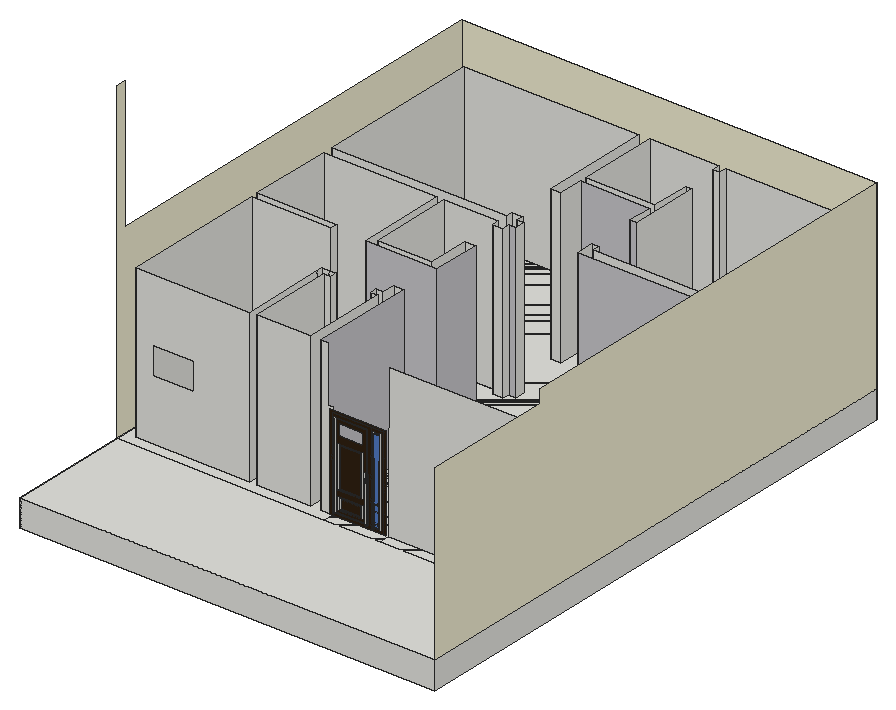
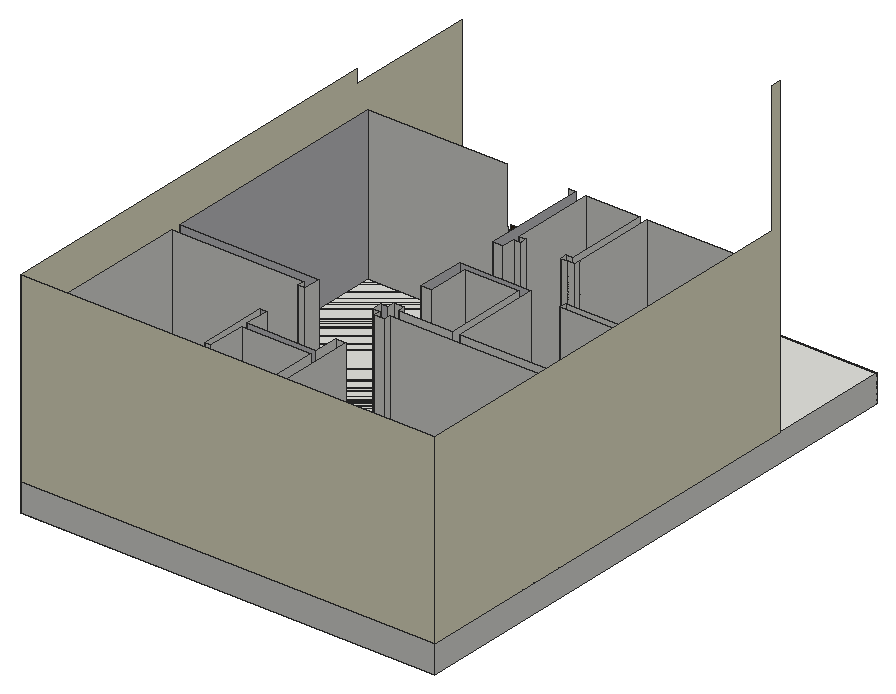
# SketchUp Ruby script. Lengths in inches.
U = 1.inch
M = Sketchup.active_model
def pt(a) = Geom::Point3d.new(a.map { |v| v * U })
def face(e, loops, mat)
  f = e.add_face(loops[0].map { |a| pt(a) })
  loops[1..].each { |l| e.add_face(l.map { |a| pt(a) }).erase! }
  f.material = f.back_material = mat if mat
  f
end
# faces: each face lists its corners as indices into pts; further lists are holes
def faces(e, pts, list, mat = nil) = list.each { |f| face(e, (f[0].is_a?(Array) ? f : [f]).map { |l| l.map { |i| pts[i] } }, mat) }
# xy, xz, yz: faces in a plane at the given z, y or x. An outline is a flat list of corners, or four numbers for a rectangle; further outlines are holes
def ring(l) = l.size == 4 ? [[l[0], l[1]], [l[2], l[1]], [l[2], l[3]], [l[0], l[3]]] : l.each_slice(2).to_a
def flat(e, list, mat, &to3) = list.each { |f| face(e, (f[0].is_a?(Array) ? f : [f]).map { |l| ring(l).map { |u, v| to3.(u, v) } }, mat) }
def xy(e, z, list, mat = nil) = flat(e, list, mat) { |x, y| [x, y, z] }
def xz(e, y, list, mat = nil) = flat(e, list, mat) { |x, z| [x, y, z] }
def yz(e, x, list, mat = nil) = flat(e, list, mat) { |y, z| [x, y, z] }
def lines(e, pts, list) = list.each { |a, b| e.add_line(pt(pts[a]), pt(pts[b])) }
# prism: a flat outline (further loops are holes) pulled along v
def prism(e, loops, v, mat = nil)
  f = face(e, loops, mat); d = Geom::Vector3d.new(v.map { |x| x * U })
  f.pushpull(f.normal.samedirection?(d) ? d.length : -d.length)
end
def box(e, o, s, mat = nil) = prism(e, [[o, [o[0] + s[0], o[1], o[2]], [o[0] + s[0], o[1] + s[1], o[2]], [o[0], o[1] + s[1], o[2]]]], [0, 0, s[2]], mat)
def at(x, y, z, deg = 0) = Geom::Transformation.translation(pt([x, y, z])) * Geom::Transformation.rotation(ORIGIN, Z_AXIS, deg.degrees)
def axes(o, x, y, z) = Geom::Transformation.new([*x, 0, *y, 0, *z, 0, *pt(o).to_a, 1])
def part(name) = M.definitions.add(name)
# library, detail: a bought-in or finely detailed component or shape, given as its bounding box
def library(name, o, s) = part(name).tap { |d| box(d.entities, o, s) }
def detail(e, o, s) = box(e.add_group.entities, o, s)
def put(e, d, t, mat = nil) = e.add_instance(d, t).tap { |i| i.material = mat if mat }
def group(e, t, mat = nil) = e.add_group.tap { |g| g.transformation = t; g.material = mat if mat }.entities
root = M.entities
M.materials.add("Lily_Blonde").color = [237, 233, 206]
M.materials.add("Panel-Opening1").color = [191, 148, 107]
M.materials.add("Stained Mahogany").color = [48, 33, 18]
M.materials.add("[Aluminum]").color = [178, 178, 178]
M.materials.add("[Metal Rusted]").color = [181, 73, 64]
M.materials.add("[Metal Silver]").color = [198, 197, 201]
M.materials.add("[Translucent Glass Blue]").color = [81, 121, 193]
c1 = part("A$C72384DA6")
p = [[1968.53,82677.18,0],[49212.62,82677.18,0],[0.02,84645.6875,0],[51181.125,84645.6875,0],[49212.62,0.02,0],[51181.125,0.02,0],
  [1968.53,0.02,0],[0.02,0.02,0]]
lines(c1.entities,p,[[0,1],[2,3],[1,4],[3,5],[0,6],[2,7],[7,6],[4,5]])
c2 = part("Floor slab")
box(c2.entities,[0,0,0],[360,480,24])
xy(root,24,[[0,125.1875,0,500.1875,360,500.1875,360,125.1875,229,125.1875,229,134.1875,351,134.1875,351,338.1875,230,338.1875,230,353.1875,236,353.1875,236,347.1875,351,347.1875,351,491.1875,236,491.1875,236,485.1875,230,485.1875,230,491.1875,170,491.1875,170,422.1875,230,422.1875,230,455.1875,236,455.1875,236,395.1875,230,395.1875,230,416.1875,170,416.1875,170,395.1875,161,395.1875,161,491.1875,9,491.1875,9,347.1875,161,347.1875,161,353.1875,170,353.1875,170,347.1875,176,347.1875,176,338.1875,170,338.1875,170,332.1875,161,332.1875,161,338.1875,114,338.1875,114,266.1875,161,266.1875,161,302.1875,170,302.1875,170,260.1875,108,260.1875,108,338.1875,9,338.1875,9,266.1875,78,266.1875,78,260.1875,9,260.1875,9,134.1875,108,134.1875,108,213.1875,120,213.1875,120,207.1875,114,207.1875,114,134.1875,161,134.1875,161,207.1875,155,207.1875,155,213.1875,161,213.1875,161,224.1875,170,224.1875,170,134.1875,180.027,134.1875,180.027,125.1875],[180.027,125.1875,180.027,134.1875,170,134.1875,170,224.1875,161,224.1875,161,213.1875,155,213.1875,155,207.1875,161,207.1875,161,134.1875,114,134.1875,114,207.1875,120,207.1875,120,213.1875,108,213.1875,108,134.1875,9,134.1875,9,260.1875,78,260.1875,78,266.1875,9,266.1875,9,338.1875,108,338.1875,108,260.1875,170,260.1875,170,302.1875,161,302.1875,161,266.1875,114,266.1875,114,338.1875,161,338.1875,161,332.1875,170,332.1875,170,338.1875,176,338.1875,176,347.1875,170,347.1875,170,353.1875,161,353.1875,161,347.1875,9,347.1875,9,491.1875,161,491.1875,161,395.1875,170,395.1875,170,416.1875,230,416.1875,230,395.1875,236,395.1875,236,455.1875,230,455.1875,230,422.1875,170,422.1875,170,491.1875,230,491.1875,230,485.1875,236,485.1875,236,491.1875,351,491.1875,351,347.1875,236,347.1875,236,353.1875,230,353.1875,230,338.1875,351,338.1875,351,134.1875,229,134.1875,229,125.1875]])
xy(root,28.183,[[218.2,130.405,224.188,131.153]])
xy(root,28.183,[[184.518,131.153,212.961,131.528],[218.2,131.153,224.188,131.528]],"Panel-Opening1")
xy(root,29.332,[[185.641,130.031,211.838,131.153]])
xy(root,29.332,[[219.323,130.592,223.066,131.528],[185.641,131.153,211.838,131.528]],"Panel-Opening1")
xy(root,32.204,[[188.447,130.031,209.031,131.153]])
xy(root,32.204,[[219.323,130.031,223.066,131.528],[188.447,131.153,209.031,131.528]],"Panel-Opening1")
xy(root,33.353,[[189.57,130.405,207.909,131.153]])
xy(root,33.353,[[219.323,130.031,223.066,131.528],[189.57,131.153,207.909,131.528]],"Panel-Opening1")
xy(root,41.012,[[189.57,130.405,207.909,131.153]])
xy(root,41.012,[[219.323,130.031,223.066,131.528],[189.57,131.153,207.909,131.528]],"Panel-Opening1")
xy(root,42.135,[[219.323,130.031,223.066,131.528]],"Panel-Opening1")
xy(root,42.161,[[188.447,130.031,209.031,131.153]])
xy(root,42.161,[[188.447,131.153,209.031,131.528]],"Panel-Opening1")
xy(root,47.905,[[188.447,130.031,209.031,131.153]])
xy(root,47.905,[[219.323,130.031,223.066,131.528],[188.447,131.153,209.031,131.528]],"Panel-Opening1")
xy(root,49.054,[[189.57,130.405,207.909,131.153]])
xy(root,49.054,[[219.323,130.031,223.066,131.528],[189.57,131.153,207.909,131.528]],"Panel-Opening1")
xy(root,61.961,[[211.838,129.656,212.961,131.528],[210.464,130.031,211.838,131.153]])
xy(root,61.961,[[210.464,131.153,211.838,131.528]],"[Aluminum]")
xy(root,62.37,[[211.693,131.528,211.713,131.715],[211.713,131.528,211.733,131.715]],"[Aluminum]")
xy(root,64.162,[[211.701,129.095,211.705,131.715],[211.721,129.095,211.724,131.715]],"[Metal Rusted]")
xy(root,64.163,[[211.709,129.095,211.713,131.715],[211.713,129.095,211.717,131.715]],"[Metal Rusted]")
xz(root,130.405,[[189.57,49.054,207.909,82.371]],"Stained Mahogany")
xz(root,130.592,[[219.323,29.332,223.066,102.093]],"[Translucent Glass Blue]")
xz(root,131.153,[[180.027,25.502,180.027,107.838,228.68,107.838,228.68,25.502,226.808,25.502,226.808,105.923,181.898,105.923,181.898,25.502],[[181.898,25.502,215.581,105.923],[184.518,28.183,212.961,103.242]],[[215.581,25.502,226.808,105.923],[218.2,28.183,224.188,103.242]],[[185.641,29.332,185.641,102.093,211.838,102.093,211.838,68.107,210.464,68.107,210.464,61.961,211.838,61.961,211.838,29.332],[188.447,47.905,209.031,83.52],[188.447,89.264,209.031,99.221],[188.447,32.204,209.031,42.161]],[189.57,33.353,207.909,41.012],
  [189.57,49.054,207.909,82.371]],"Stained Mahogany")
xz(root,131.528,[[184.518,28.183,184.518,103.242,212.961,103.242,212.961,68.107,211.838,68.107,211.838,102.093,185.641,102.093,185.641,29.332,211.838,29.332,211.838,61.961,212.961,61.961,212.961,28.183],[[218.2,28.183,224.188,103.242],[219.323,49.054,223.066,82.371],[219.323,33.353,223.066,41.012],[219.323,90.413,223.066,98.072],[219.323,42.135,223.066,47.905],[219.323,83.52,223.066,89.264],[219.323,99.221,223.066,102.093],[219.323,29.332,223.066,32.204]],[[188.447,32.204,209.031,42.161],[189.57,33.353,207.909,41.012]],[[188.447,47.905,209.031,83.52],[189.57,49.054,207.909,82.371]]],"Panel-Opening1")
xz(root,131.528,[[[210.464,61.961,212.961,68.107],[211.713,65.58,211.776,65.583,211.838,65.589,211.9,65.599,211.961,65.614,212.022,65.633,212.081,65.655,212.138,65.682,212.193,65.712,212.247,65.746,212.298,65.784,212.347,65.825,212.392,65.869,212.435,65.916,212.475,65.965,212.512,66.018,212.545,66.072,212.575,66.129,212.601,66.188,212.623,66.248,212.641,66.31,212.656,66.372,212.666,66.436,212.672,66.5,212.674,66.564,212.672,66.629,212.666,66.693,212.656,66.756,212.641,66.819,212.623,66.88,212.601,66.941,212.575,66.999,212.545,67.056,212.512,67.111,212.475,67.163,212.435,67.213,212.392,67.26,212.347,67.304,212.298,67.345,212.247,67.382,212.193,67.416,212.138,67.447,212.081,67.473,212.022,67.496,211.961,67.514,211.9,67.529,211.838,67.54,211.776,67.546,211.713,67.548,211.65,67.546,211.587,67.54,211.525,67.529,211.464,67.514,211.404,67.496,211.345,67.473,211.287,67.447,211.232,67.416,211.179,67.382,211.127,67.345,211.079,67.304,211.033,67.26,210.99,67.213,210.95,67.163,210.913,67.111,210.88,67.056,210.85,66.999,210.824,66.941,210.802,66.88,210.784,66.819,210.77,66.756,210.759,66.693,210.753,66.629,210.751,66.564,210.753,66.5,210.759,66.436,210.77,66.372,210.784,66.31,210.802,66.248,210.824,66.188,210.85,66.129,210.88,66.072,210.913,66.018,210.95,65.965,210.99,65.916,211.033,65.869,211.079,65.825,211.127,65.784,211.179,65.746,211.232,65.712,211.287,65.682,211.345,65.655,211.404,65.633,211.464,65.614,211.525,65.599,211.587,65.589,211.65,65.583],[211.693,62.37,211.733,62.37,211.753,62.372,211.773,62.376,211.792,62.38,211.811,62.386,211.83,62.394,211.838,62.397,211.849,62.402,211.866,62.412,211.883,62.423,211.9,62.435,211.915,62.448,211.93,62.462,211.944,62.477,211.968,62.509,211.979,62.527,211.988,62.545,211.997,62.564,212.004,62.583,212.014,62.623,212.017,62.643,212.019,62.664,212.02,62.684,212.02,64.101,212.019,64.122,212.017,64.142,212.014,64.163,212.004,64.203,211.997,64.222,211.988,64.241,211.979,64.259,211.968,64.276,211.956,64.293,211.944,64.309,211.93,64.324,211.915,64.338,211.9,64.351,211.883,64.363,211.866,64.374,211.849,64.383,211.838,64.388,211.83,64.392,211.811,64.399,211.792,64.405,211.773,64.41,211.753,64.413,211.733,64.415,211.713,64.416,211.693,64.415,211.673,64.413,211.653,64.41,211.633,64.405,211.614,64.399,211.595,64.392,211.559,64.374,211.542,64.363,211.526,64.351,211.51,64.338,211.495,64.324,211.482,64.309,211.469,64.293,211.457,64.276,211.447,64.259,211.437,64.241,211.429,64.222,211.422,64.203,211.416,64.183,211.411,64.163,211.408,64.142,211.406,64.122,211.405,64.101,211.405,62.684,211.406,62.664,211.408,62.643,211.411,62.623,211.416,62.603,211.422,62.583,211.429,62.564,211.437,62.545,211.457,62.509,211.469,62.493,211.482,62.477,211.495,62.462,211.51,62.448,211.526,62.435,211.542,62.423,211.559,62.412,211.577,62.402,211.595,62.394,211.614,62.386,211.633,62.38,211.673,62.372]]],"[Aluminum]")
xz(root,131.715,[[[211.693,62.37,211.673,62.372,211.633,62.38,211.614,62.386,211.595,62.394,211.577,62.402,211.559,62.412,211.542,62.423,211.526,62.435,211.51,62.448,211.495,62.462,211.482,62.477,211.469,62.493,211.457,62.509,211.437,62.545,211.429,62.564,211.422,62.583,211.416,62.603,211.411,62.623,211.408,62.643,211.406,62.664,211.405,62.684,211.405,64.101,211.406,64.122,211.408,64.142,211.411,64.163,211.416,64.183,211.422,64.203,211.429,64.222,211.437,64.241,211.447,64.259,211.457,64.276,211.469,64.293,211.482,64.309,211.495,64.324,211.51,64.338,211.526,64.351,211.542,64.363,211.559,64.374,211.595,64.392,211.614,64.399,211.633,64.405,211.653,64.41,211.673,64.413,211.693,64.415,211.713,64.416,211.733,64.415,211.753,64.413,211.773,64.41,211.792,64.405,211.811,64.399,211.83,64.392,211.838,64.388,211.849,64.383,211.866,64.374,211.883,64.363,211.9,64.351,211.915,64.338,211.93,64.324,211.944,64.309,211.956,64.293,211.968,64.276,211.979,64.259,211.988,64.241,211.997,64.222,212.004,64.203,212.014,64.163,212.017,64.142,212.019,64.122,212.02,64.101,212.02,62.684,212.019,62.664,212.017,62.643,212.014,62.623,212.004,62.583,211.997,62.564,211.988,62.545,211.979,62.527,211.968,62.509,211.944,62.477,211.93,62.462,211.915,62.448,211.9,62.435,211.883,62.423,211.866,62.412,211.849,62.402,211.838,62.397,211.83,62.394,211.811,62.386,211.792,62.38,211.773,62.376,211.753,62.372,211.733,62.37],[211.652,62.916,211.773,62.916,211.773,64.105,211.772,64.109,211.772,64.113,211.77,64.121,211.768,64.125,211.767,64.128,211.765,64.132,211.763,64.135,211.761,64.139,211.75,64.15,211.746,64.152,211.743,64.154,211.739,64.156,211.736,64.158,211.732,64.159,211.728,64.161,211.724,64.162,211.721,64.162,211.717,64.163,211.709,64.163,211.705,64.162,211.701,64.162,211.697,64.161,211.693,64.159,211.689,64.158,211.686,64.156,211.682,64.154,211.676,64.15,211.673,64.147,211.67,64.145,211.667,64.142,211.665,64.139,211.662,64.135,211.66,64.132,211.658,64.128,211.657,64.125,211.655,64.121,211.653,64.113,211.653,64.109,211.652,64.105]]],"[Aluminum]")
xz(root,134.1875,[[[9,24,108,156],[24,77,60,101]],[114,24,161,156],[170,24,170,156,176,156,176,108,180.027,108,180.027,24],[229,24,229,108,230,108,230,156,351,156,351,24]])
xz(root,207.1875,[[114,24,120,156],[155,24,161,156]])
xz(root,213.1875,[[108,24,114,156],[114,24,120,156],[155,24,161,156]])
xz(root,224.1875,[[161,24,170,156]])
xz(root,260.1875,[[9,24,78,156]])
xz(root,260.1875,[[108,24,170,156]],"[Metal Silver]")
xz(root,266.1875,[[9,24,78,156],[114,24,161,156]])
xz(root,302.1875,[[161,24,170,156]])
xz(root,332.1875,[[161,24,170,156]])
xz(root,338.1875,[[9,24,108,156],[114,24,161,156]])
xz(root,338.1875,[[170,24,176,156],[230,24,351,156]],"[Metal Silver]")
xz(root,347.1875,[[9,24,161,156],[170,24,176,156],[236,24,351,156]])
xz(root,353.1875,[[161,24,170,156],[230,24,236,156]])
xz(root,395.1875,[[161,24,170,156]])
xz(root,395.1875,[[230,24,236,156]],"[Metal Silver]")
xz(root,416.1875,[[170,24,230,156]],"[Metal Silver]")
xz(root,422.1875,[[170,24,230,156]])
xz(root,455.1875,[[230,24,236,156]])
xz(root,485.1875,[[230,24,236,156]])
xz(root,491.1875,[[9,24,161,156],[170,24,230,156],[236,24,351,156]])
xz(root,500.1875,[[0,24,360,185]],"Lily_Blonde")
yz(root,0,[[125.1875,24,125.1875,298,134.1875,298,134.1875,185,500.1875,185,500.1875,24]],"Lily_Blonde")
yz(root,9,[[134.1875,24,260.1875,156],[266.1875,24,338.1875,156],[347.1875,24,491.1875,156]])
yz(root,78,[[260.1875,24,266.1875,156]])
yz(root,108,[[134.1875,24,207.1875,156],[207.1875,24,213.1875,156],[260.1875,24,338.1875,156]])
yz(root,114,[[134.1875,24,207.1875,156],[266.1875,24,338.1875,156]])
yz(root,120,[[207.1875,24,213.1875,156]])
yz(root,155,[[207.1875,24,213.1875,156]])
yz(root,161,[[134.1875,24,207.1875,156],[213.1875,24,224.1875,156],[266.1875,24,302.1875,156],[332.1875,24,338.1875,156],[347.1875,24,353.1875,156],
  [395.1875,24,491.1875,156]])
yz(root,170,[[332.1875,24,338.1875,156],[347.1875,24,353.1875,156],[395.1875,24,416.1875,156],[422.1875,24,491.1875,156]])
yz(root,170,[[134.1875,24,224.1875,156],[260.1875,24,302.1875,156]],"[Metal Silver]")
yz(root,176,[[338.1875,24,347.1875,156]])
yz(root,184.518,[[129.656,28.183,131.153,103.242]])
yz(root,184.518,[[131.153,28.183,131.528,103.242]],"Panel-Opening1")
yz(root,185.641,[[130.031,29.332,131.153,102.093]])
yz(root,185.641,[[131.153,29.332,131.528,102.093]],"Panel-Opening1")
yz(root,188.447,[[130.031,32.204,131.153,42.161],[130.031,47.905,131.153,83.52]])
yz(root,188.447,[[131.153,32.204,131.528,42.161],[131.153,47.905,131.528,83.52]],"Panel-Opening1")
yz(root,189.57,[[130.405,33.353,131.153,41.012],[130.405,49.054,131.153,82.371]])
yz(root,189.57,[[131.153,33.353,131.528,41.012],[131.153,49.054,131.528,82.371]],"Panel-Opening1")
yz(root,207.909,[[130.405,33.353,131.153,41.012],[130.405,49.054,131.153,82.371]])
yz(root,207.909,[[131.153,33.353,131.528,41.012],[131.153,49.054,131.528,82.371]],"Panel-Opening1")
yz(root,209.031,[[130.031,32.204,131.153,42.161],[130.031,47.905,131.153,83.52]])
yz(root,209.031,[[131.153,32.204,131.528,42.161],[131.153,47.905,131.528,83.52]],"Panel-Opening1")
yz(root,210.464,[[130.031,61.961,131.153,68.107]])
yz(root,210.464,[[131.153,61.961,131.528,68.107]],"[Aluminum]")
yz(root,211.405,[[131.528,62.684,131.715,64.101]],"[Aluminum]")
yz(root,211.838,[[130.031,29.332,131.153,61.961]])
yz(root,211.838,[[131.153,29.332,131.528,61.961]],"Panel-Opening1")
yz(root,212.02,[[131.528,62.684,131.715,64.101]],"[Aluminum]")
yz(root,212.961,[[131.153,28.183,131.528,61.961]],"Panel-Opening1")
yz(root,212.961,[[131.153,61.961,131.528,68.107]],"[Aluminum]")
yz(root,218.2,[[130.405,28.183,131.153,103.242]])
yz(root,218.2,[[131.153,28.183,131.528,103.242]],"Panel-Opening1")
yz(root,219.323,[[130.592,32.204,131.153,33.353]])
yz(root,219.323,[[130.592,29.332,131.528,32.204],[130.592,33.353,131.528,41.012],[130.592,42.135,131.528,47.905],[130.592,49.054,131.528,82.371]],"Panel-Opening1")
yz(root,223.066,[[130.592,32.204,131.153,33.353]])
yz(root,223.066,[[130.592,29.332,131.528,32.204],[130.592,33.353,131.528,41.012],[130.592,42.135,131.528,47.905],[130.592,49.054,131.528,82.371]],"Panel-Opening1")
yz(root,224.188,[[130.405,28.183,131.153,103.242]])
yz(root,224.188,[[131.153,28.183,131.528,103.242]],"Panel-Opening1")
yz(root,230,[[338.1875,24,353.1875,156],[395.1875,24,416.1875,156],[422.1875,24,455.1875,156],[485.1875,24,491.1875,156]])
yz(root,236,[[347.1875,24,353.1875,156],[395.1875,24,455.1875,156],[485.1875,24,491.1875,156]])
yz(root,351,[[347.1875,24,491.1875,156]])
yz(root,351,[[134.1875,24,338.1875,156]],"[Metal Silver]")
yz(root,360,[[20.75,24,500.1875,24,500.1875,185,134.1875,185,134.1875,173,20.75,173]],"Lily_Blonde")
p = [[211.559,131.528,62.412],[211.542,131.528,62.423],[211.542,131.715,62.423],[211.559,131.715,62.412],[211.526,131.528,62.435],[211.526,131.715,62.435],
  [211.51,131.528,62.448],[211.51,131.715,62.448],[211.495,131.528,62.462],[211.495,131.715,62.462],[211.653,131.528,62.376],[211.633,131.528,62.38],
  [211.633,131.715,62.38],[211.653,131.715,62.376],[211.614,131.528,62.386],[211.614,131.715,62.386],[211.595,131.528,62.394],[211.595,131.715,62.394],
  [211.577,131.528,62.402],[211.577,131.715,62.402],[211.693,131.528,62.37],[211.673,131.528,62.372],[211.673,131.715,62.372],[211.693,131.715,62.37],
  [211.753,131.528,62.372],[211.733,131.528,62.37],[211.733,131.715,62.37],[211.753,131.715,62.372],[211.773,131.528,62.376],[211.773,131.715,62.376],
  [211.792,131.528,62.38],[211.792,131.715,62.38],[211.811,131.528,62.386],[211.811,131.715,62.386],[211.83,131.528,62.394],[211.83,131.715,62.394],
  [211.838,131.528,62.397],[211.838,131.715,62.397],[211.849,131.528,62.402],[211.849,131.715,62.402],[211.866,131.528,62.412],[211.866,131.715,62.412],
  [211.883,131.528,62.423],[211.883,131.715,62.423],[211.9,131.528,62.435],[211.9,131.715,62.435],[211.915,131.528,62.448],[211.915,131.715,62.448],
  [211.93,131.528,62.462],[211.93,131.715,62.462],[211.457,131.528,62.509],[211.447,131.528,62.527],[211.447,131.715,62.527],[211.457,131.715,62.509],
  [211.437,131.528,62.545],[211.437,131.715,62.545],[211.429,131.528,62.564],[211.429,131.715,62.564],[211.482,131.528,62.477],[211.482,131.715,62.477],
  [211.469,131.528,62.493],[211.469,131.715,62.493],[211.944,131.528,62.477],[211.944,131.715,62.477],[211.956,131.528,62.493],[211.956,131.715,62.493],
  [211.968,131.528,62.509],[211.968,131.715,62.509],[211.979,131.528,62.527],[211.979,131.715,62.527],[211.988,131.528,62.545],[211.988,131.715,62.545],
  [211.997,131.528,62.564],[211.997,131.715,62.564],[211.422,131.528,62.583],[211.422,131.715,62.583],[211.416,131.528,62.603],[211.416,131.715,62.603],
  [211.411,131.528,62.623],[211.411,131.715,62.623],[211.408,131.528,62.643],[211.408,131.715,62.643],[211.406,131.528,62.664],[211.406,131.715,62.664],
  [212.004,131.528,62.583],[212.004,131.715,62.583],[212.009,131.528,62.603],[212.009,131.715,62.603],[212.014,131.528,62.623],[212.014,131.715,62.623],
  [212.017,131.528,62.643],[212.017,131.715,62.643],[212.019,131.528,62.664],[212.019,131.715,62.664],[211.405,131.528,62.684],[211.405,131.715,62.684],
  [212.02,131.528,62.684],[212.02,131.715,62.684],[211.75,131.715,64.15],[211.75,129.095,64.15],[211.753,129.095,64.147],[211.753,131.715,64.147],
  [211.676,131.715,64.15],[211.676,129.095,64.15],[211.679,129.095,64.152],[211.679,131.715,64.152],[211.746,131.715,64.152],[211.746,129.095,64.152],
  [211.405,131.528,64.101],[211.406,131.528,64.122],[211.406,131.715,64.122],[211.405,131.715,64.101],[211.408,131.528,64.142],[211.408,131.715,64.142],
  [211.411,131.528,64.163],[211.411,131.715,64.163],[212.019,131.528,64.122],[212.02,131.528,64.101],[212.02,131.715,64.101],[212.019,131.715,64.122],
  [212.017,131.528,64.142],[212.017,131.715,64.142],[212.014,131.528,64.163],[212.014,131.715,64.163],[211.743,131.715,64.154],[211.743,129.095,64.154],
  [211.682,129.095,64.154],[211.682,131.715,64.154],[211.686,129.095,64.156],[211.686,131.715,64.156],[211.739,131.715,64.156],[211.739,129.095,64.156],
  [211.689,129.095,64.158],[211.689,131.715,64.158],[211.736,131.715,64.158],[211.736,129.095,64.158],[211.732,131.715,64.159],[211.732,129.095,64.159],
  [211.693,129.095,64.159],[211.693,131.715,64.159],[211.728,131.715,64.161],[211.728,129.095,64.161],[211.697,129.095,64.161],[211.697,131.715,64.161],
  [211.701,129.095,64.162],[211.701,131.715,64.162],[211.724,131.715,64.162],[211.724,129.095,64.162],[211.705,131.715,64.162],[211.705,129.095,64.162],
  [211.709,129.095,64.163],[211.709,131.715,64.163],[211.717,131.715,64.163],[211.717,129.095,64.163],[211.721,129.095,64.162],[211.721,131.715,64.162],
  [211.411,129.282,64.163],[211.416,129.282,64.183],[211.416,131.528,64.183],[211.422,129.282,64.203],[211.422,131.528,64.203],[211.429,129.282,64.222],
  [211.429,131.528,64.222],[211.437,129.282,64.241],[211.437,131.528,64.241],[211.447,129.282,64.259],[211.447,131.528,64.259],[212.009,131.528,64.183],
  [212.009,129.282,64.183],[212.014,129.282,64.163],[212.004,131.528,64.203],[212.004,129.282,64.203],[211.997,131.528,64.222],[211.997,129.282,64.222],
  [211.988,131.528,64.241],[211.988,129.282,64.241],[211.979,131.528,64.259],[211.979,129.282,64.259],[211.416,131.715,64.183],[211.422,131.715,64.203],
  [211.429,131.715,64.222],[211.437,131.715,64.241],[211.447,131.715,64.259],[212.009,131.715,64.183],[212.004,131.715,64.203],[211.997,131.715,64.222],
  [211.988,131.715,64.241],[211.979,131.715,64.259],[211.457,129.282,64.276],[211.457,131.528,64.276],[211.469,129.282,64.293],[211.469,131.528,64.293],
  [211.482,129.282,64.309],[211.482,131.528,64.309],[211.495,129.282,64.324],[211.495,131.528,64.324],[211.51,129.282,64.338],[211.51,131.528,64.338],
  [211.526,129.282,64.351],[211.526,131.528,64.351],[211.944,131.528,64.309],[211.944,129.282,64.309],[211.956,129.282,64.293],[211.956,131.528,64.293],
  [211.93,131.528,64.324],[211.93,129.282,64.324],[211.915,131.528,64.338],[211.915,129.282,64.338],[211.9,131.528,64.351],[211.9,129.282,64.351],
  [211.968,131.528,64.276],[211.968,129.282,64.276],[211.457,131.715,64.276],[211.469,131.715,64.293],[211.482,131.715,64.309],[211.495,131.715,64.324],
  [211.51,131.715,64.338],[211.526,131.715,64.351],[211.956,131.715,64.293],[211.944,131.715,64.309],[211.93,131.715,64.324],[211.915,131.715,64.338],
  [211.9,131.715,64.351],[211.968,131.715,64.276],[211.542,129.282,64.363],[211.542,131.528,64.363],[211.559,129.282,64.374],[211.559,131.528,64.374],
  [211.577,129.282,64.383],[211.577,131.528,64.383],[211.595,129.282,64.392],[211.595,131.528,64.392],[211.614,129.282,64.399],[211.614,131.528,64.399],
  [211.633,129.282,64.405],[211.633,131.528,64.405],[211.653,129.282,64.41],[211.653,131.528,64.41],[211.673,129.282,64.413],[211.673,131.528,64.413],
  [211.693,129.282,64.415],[211.693,131.528,64.415],[211.733,131.528,64.415],[211.733,129.282,64.415],[211.753,129.282,64.413],[211.753,131.528,64.413],
  [211.713,129.282,64.416],[211.713,131.528,64.416],[211.849,131.528,64.383],[211.849,129.282,64.383],[211.866,129.282,64.374],[211.866,131.528,64.374],
  [211.838,131.528,64.388],[211.838,129.282,64.388],[211.83,131.528,64.392],[211.83,129.282,64.392],[211.811,131.528,64.399],[211.811,129.282,64.399],
  [211.792,131.528,64.405],[211.792,129.282,64.405],[211.773,131.528,64.41],[211.773,129.282,64.41],[211.883,131.528,64.363],[211.883,129.282,64.363],
  [211.542,131.715,64.363],[211.559,131.715,64.374],[211.577,131.715,64.383],[211.595,131.715,64.392],[211.614,131.715,64.399],[211.633,131.715,64.405],
  [211.653,131.715,64.41],[211.673,131.715,64.413],[211.753,131.715,64.413],[211.733,131.715,64.415],[211.693,131.715,64.415],[211.713,131.715,64.416],
  [211.866,131.715,64.374],[211.849,131.715,64.383],[211.838,131.715,64.388],[211.83,131.715,64.392],[211.811,131.715,64.399],[211.792,131.715,64.405],
  [211.773,131.715,64.41],[211.883,131.715,64.363]]
faces(root,p,[[0,1,2,3],[1,4,5,2],[4,6,7,5],[6,8,9,7],[10,11,12,13],[11,14,15,12],[14,16,17,15],[16,18,19,17],
  [18,0,3,19],[20,21,22,23],[24,25,26,27],[21,10,13,22],[28,24,27,29],[30,28,29,31],[32,30,31,33],[34,32,33,35],
  [36,34,35,37],[38,36,37,39],[40,38,39,41],[42,40,41,43],[44,42,43,45],[46,44,45,47],[48,46,47,49],[50,51,52,53],
  [51,54,55,52],[54,56,57,55],[8,58,59,9],[58,60,61,59],[60,50,53,61],[62,48,49,63],[64,62,63,65],[66,64,65,67],
  [68,66,67,69],[70,68,69,71],[72,70,71,73],[56,74,75,57],[74,76,77,75],[76,78,79,77],[78,80,81,79],[80,82,83,81],
  [84,72,73,85],[86,84,85,87],[88,86,87,89],[90,88,89,91],[92,90,91,93],[82,94,95,83],[96,92,93,97],[108,109,110,111],
  [109,112,113,110],[112,114,115,113],[116,117,118,119],[120,116,119,121],[122,120,121,123],[114,158,178,115],[158,160,179,178],[160,162,180,179],
  [162,164,181,180],[164,166,182,181],[167,122,123,183],[170,167,183,184],[172,170,184,185],[174,172,185,186],[176,174,186,187],[166,189,212,182],
  [189,191,213,212],[191,193,214,213],[193,195,215,214],[195,197,216,215],[197,199,217,216],[200,203,218,219],[204,200,219,220],[206,204,220,221],
  [208,206,221,222],[210,176,187,223],[203,210,223,218],[199,225,264,217],[225,227,265,264],[227,229,266,265],[229,231,267,266],[231,233,268,267],
  [233,235,269,268],[235,237,270,269],[237,239,271,270],[242,245,272,273],[239,241,274,271],[241,247,275,274],[247,242,273,275],[248,251,276,277],
  [252,248,277,278],[254,252,278,279],[256,254,279,280],[258,256,280,281],[260,258,281,282],[245,260,282,272],[262,208,222,283],[251,262,283,276]],"[Aluminum]")
faces(root,p,[[98,99,100,101],[102,103,104,105],[106,107,99,98],[124,125,107,106],[105,104,126,127],[127,126,128,129],[130,131,125,124],[129,128,132,133],
  [134,135,131,130],[136,137,135,134],[133,132,138,139],[140,141,137,136],[139,138,142,143],[143,142,144,145],[146,147,141,140],[148,149,150,151],
  [152,153,154,155]],"[Metal Rusted]")
faces(root,p,[[114,156,157,158],[158,157,159,160],[160,159,161,162],[162,161,163,164],[164,163,165,166],[167,168,169,122],[170,171,168,167],[172,173,171,170],
  [174,175,173,172],[176,177,175,174],[166,165,188,189],[189,188,190,191],[191,190,192,193],[193,192,194,195],[195,194,196,197],[197,196,198,199],
  [200,201,202,203],[204,205,201,200],[206,207,205,204],[208,209,207,206],[210,211,177,176],[203,202,211,210],[199,198,224,225],[225,224,226,227],
  [227,226,228,229],[229,228,230,231],[231,230,232,233],[233,232,234,235],[235,234,236,237],[237,236,238,239],[239,238,240,241],[242,243,244,245],
  [241,240,246,247],[247,246,243,242],[248,249,250,251],[252,253,249,248],[254,255,253,252],[256,257,255,254],[258,259,257,256],[260,261,259,258],
  [245,244,261,260],[262,263,209,208],[251,250,263,262]])
put(root,c1,axes([228.68,131.15,25.5],[-0.00095,0,0],[0,0,0.00097],[0,-0.9506,0]))
put(root,c2,at(0,20.1875,0))
